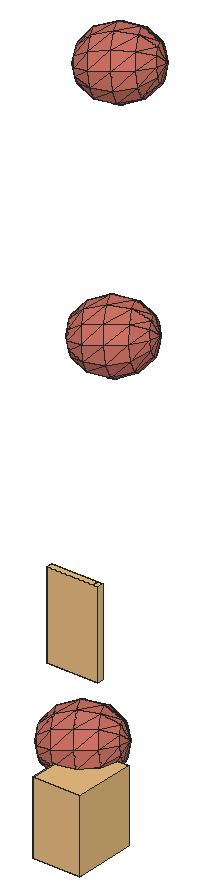
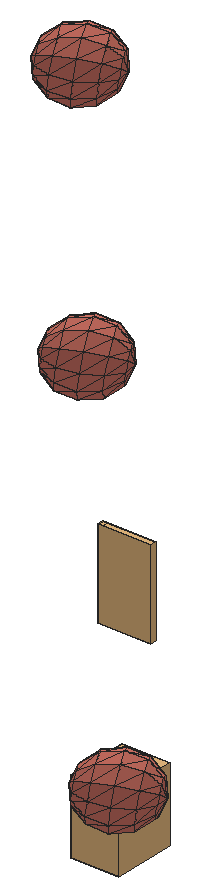
# SketchUp Ruby script. Lengths in inches.
U = 1.inch
M = Sketchup.active_model
def pt(a) = Geom::Point3d.new(a.map { |v| v * U })
def face(e, loops, mat)
  f = e.add_face(loops[0].map { |a| pt(a) })
  loops[1..].each { |l| e.add_face(l.map { |a| pt(a) }).erase! }
  f.material = f.back_material = mat if mat
  f
end
# faces: each face lists its corners as indices into pts; further lists are holes
def faces(e, pts, list, mat = nil) = list.each { |f| face(e, (f[0].is_a?(Array) ? f : [f]).map { |l| l.map { |i| pts[i] } }, mat) }
# xy, xz, yz: faces in a plane at the given z, y or x. An outline is a flat list of corners, or four numbers for a rectangle; further outlines are holes
def ring(l) = l.size == 4 ? [[l[0], l[1]], [l[2], l[1]], [l[2], l[3]], [l[0], l[3]]] : l.each_slice(2).to_a
def flat(e, list, mat, &to3) = list.each { |f| face(e, (f[0].is_a?(Array) ? f : [f]).map { |l| ring(l).map { |u, v| to3.(u, v) } }, mat) }
def xy(e, z, list, mat = nil) = flat(e, list, mat) { |x, y| [x, y, z] }
def xz(e, y, list, mat = nil) = flat(e, list, mat) { |x, z| [x, y, z] }
def yz(e, x, list, mat = nil) = flat(e, list, mat) { |y, z| [x, y, z] }
def lines(e, pts, list) = list.each { |a, b| e.add_line(pt(pts[a]), pt(pts[b])) }
# prism: a flat outline (further loops are holes) pulled along v
def prism(e, loops, v, mat = nil)
  f = face(e, loops, mat); d = Geom::Vector3d.new(v.map { |x| x * U })
  f.pushpull(f.normal.samedirection?(d) ? d.length : -d.length)
end
def box(e, o, s, mat = nil) = prism(e, [[o, [o[0] + s[0], o[1], o[2]], [o[0] + s[0], o[1] + s[1], o[2]], [o[0], o[1] + s[1], o[2]]]], [0, 0, s[2]], mat)
def at(x, y, z, deg = 0) = Geom::Transformation.translation(pt([x, y, z])) * Geom::Transformation.rotation(ORIGIN, Z_AXIS, deg.degrees)
def axes(o, x, y, z) = Geom::Transformation.new([*x, 0, *y, 0, *z, 0, *pt(o).to_a, 1])
def part(name) = M.definitions.add(name)
# library, detail: a bought-in or finely detailed component or shape, given as its bounding box
def library(name, o, s) = part(name).tap { |d| box(d.entities, o, s) }
def detail(e, o, s) = box(e.add_group.entities, o, s)
def put(e, d, t, mat = nil) = e.add_instance(d, t).tap { |i| i.material = mat if mat }
def group(e, t, mat = nil) = e.add_group.tap { |g| g.transformation = t; g.material = mat if mat }.entities
root = M.entities
M.materials.add("green").color = [174, 139, 102]
M.materials.add("vio").color = [206, 114, 100]
c1 = part("3DGeom~236_Defintion")
p = [[-0.24,-111.46,-482.47],[-247.71,40.8125,-431.68],[-3.37,-2.64,-500],[241.88,-45.39,-434.35],[50.53,96.35,-484.34],[-154.36,212.27,-404.56],
  [147.01,158.99,-439.69],[12.76,320.76,-327.23],[59.09,-200.9375,-436.46],[-242.29,-147.66,-401.32],[260.24,168.49,-378.02],[208.87,337.23,-220.41],
  [208.87,337.23,-220.41],[-139.53,-302.65,-321.625],[158.71,-247.11,-374.29],[271.93,-237.61,-312.62],[368.42,-174.96,-267.97],[422.32,-75.98,-252.31],
  [419.18,32.84,-269.83],[359.86,122.32,-315.85],[-242.29,-147.66,-401.32],[-425.68,73.33,-247.69],[-247.71,40.8125,-431.68],[-425.68,73.33,-247.69],
  [-317.89,271.31,-216.37],[-317.89,271.31,-216.37],[-154.36,212.27,-404.56],[-317.89,271.31,-216.37],[-124.92,396.59,-127.08],[-154.36,212.27,-404.56],
  [12.76,320.76,-327.23],[-139.53,-302.65,-321.625],[-419.42,-144.29,-212.64],[-242.29,-147.66,-401.32],[-242.29,-147.66,-401.32],[-425.68,73.33,-247.69],
  [260.24,168.49,-378.02],[381.41,257.26,-112.72],[359.86,122.32,-315.85],[260.24,168.49,-378.02],[208.87,337.23,-220.41],[33.01,-382.62,-213.94],
  [271.93,-237.61,-312.62],[33.01,-382.62,-213.94],[158.71,-247.11,-374.29],[12.76,320.76,-327.23],[101.53,415.61,-3.73],[12.76,320.76,-327.23],
  [208.87,337.23,-220.41],[33.01,-382.62,-213.94],[-300.77,-323.26,-120.61],[-139.53,-302.65,-321.625],[-139.53,-302.65,-321.625],[-300.77,-323.26,-120.61],
  [359.86,122.32,-315.85],[484.17,102.27,-33.02],[419.18,32.84,-269.83],[359.86,122.32,-315.85],[271.93,-237.61,-312.62],[229.12,-366.15,-107.12],
  [33.01,-382.62,-213.94],[368.42,-174.96,-267.97],[229.12,-366.15,-107.12],[271.93,-237.61,-312.62],[419.18,32.84,-269.83],[489.59,-86.2,-2.67],
  [419.18,32.84,-269.83],[422.32,-75.98,-252.31],[368.42,-174.96,-267.97],[396.24,-257.66,-29.79],[229.12,-366.15,-107.12],[422.32,-75.98,-252.31],
  [368.42,-174.96,-267.97],[422.32,-75.98,-252.31],[-489.59,86.2,2.67],[-425.68,73.33,-247.69],[-425.68,73.33,-247.69],[-396.24,257.66,29.79],
  [-425.68,73.33,-247.69],[-396.24,257.66,29.79],[-317.89,271.31,-216.37],[208.87,337.23,-220.41],[300.77,323.26,120.61],[381.41,257.26,-112.72],
  [208.87,337.23,-220.41],[300.77,323.26,120.61],[-396.24,257.66,29.79],[-229.12,366.15,107.12],[33.01,-382.62,-213.94],[-101.53,-415.61,3.73],
  [-300.77,-323.26,-120.61],[33.01,-382.62,-213.94],[-484.17,-102.27,33.02],[-33.01,382.62,213.94],[-381.41,-257.26,112.72],[-300.77,-323.26,-120.61],
  [-381.41,-257.26,112.72],[419.42,144.29,212.64],[300.77,323.26,120.61],[124.92,-396.59,127.08],[396.24,-257.66,-29.79],[425.68,-73.33,247.69],
  [396.24,-257.66,-29.79],[317.89,-271.31,216.37],[317.89,-271.31,216.37],[139.53,302.65,321.625],[139.53,302.65,321.625],[300.77,323.26,120.61],
  [-422.32,75.98,252.31],[-368.42,174.96,267.97],[-396.24,257.66,29.79],[-208.87,-337.23,220.41],[-381.41,-257.26,112.72],[-396.24,257.66,29.79],
  [-271.93,237.61,312.62],[-396.24,257.66,29.79],[-271.93,237.61,312.62],[-229.12,366.15,107.12],[-419.18,-32.84,269.83],[-271.93,237.61,312.62],
  [-158.71,247.11,374.29],[-158.71,247.11,374.29],[-208.87,-337.23,220.41],[-359.86,-122.32,315.85],[242.29,147.66,401.32],[139.53,302.65,321.625],
  [-12.76,-320.76,327.23],[317.89,-271.31,216.37],[247.71,-40.8125,431.68],[247.71,-40.8125,431.68],[-33.01,382.62,213.94],[-158.71,247.11,374.29],
  [-59.09,200.94,436.46],[-33.01,382.62,213.94],[139.53,302.65,321.625],[317.89,-271.31,216.37],[154.36,-212.27,404.56],[425.68,-73.33,247.69],
  [154.36,-212.27,404.56],[317.89,-271.31,216.37],[-208.87,-337.23,220.41],[-260.24,-168.49,378.02],[-12.76,-320.76,327.23],[-260.24,-168.49,378.02],
  [-208.87,-337.23,220.41],[425.68,-73.33,247.69],[247.71,-40.8125,431.68],[-422.32,75.98,252.31],[-419.18,-32.84,269.83],[-241.88,45.39,434.35],
  [-368.42,174.96,267.97],[-422.32,75.98,252.31],[-271.93,237.61,312.62],[-368.42,174.96,267.97],[-419.18,-32.84,269.83],[-359.86,-122.32,315.85],
  [-271.93,237.61,312.62],[-359.86,-122.32,315.85],[-260.24,-168.49,378.02],[139.53,302.65,321.625],[0.24,111.46,482.47],[139.53,302.65,321.625],
  [242.29,147.66,401.32],[-12.76,-320.76,327.23],[-147.01,-158.99,439.69],[-260.24,-168.49,378.02],[-12.76,-320.76,327.23],[-260.24,-168.49,378.02],
  [242.29,147.66,401.32],[3.37,2.64,500],[242.29,147.66,401.32],[-50.53,-96.35,484.34]]
faces(c1.entities,p,[[0,1,2],[0,2,3],[2,4,3],[2,1,5],[2,5,4],[4,6,3],[4,5,7],[4,7,6],
  [8,9,0],[8,0,3],[0,9,1],[6,10,3],[6,7,11],[6,12,10],[8,13,9],[14,13,8],
  [14,8,3],[15,14,3],[16,15,3],[17,16,3],[18,17,3],[19,18,3],[10,19,3],[20,21,22],
  [1,23,24],[1,25,5],[26,27,28],[29,28,30],[31,32,33],[34,32,35],[36,37,38],[39,40,37],
  [14,41,13],[42,43,44],[45,28,46],[47,46,48],[49,50,51],[52,53,32],[54,55,56],[57,37,55],
  [58,59,60],[61,62,63],[64,55,65],[66,65,67],[68,69,70],[71,69,72],[73,65,69],[32,74,75],
  [76,74,77],[78,79,80],[81,82,83],[84,46,85],[27,86,87],[27,87,28],[88,89,90],[59,89,91],
  [53,92,32],[32,92,74],[28,87,93],[28,93,46],[89,94,95],[53,96,92],[37,97,55],[37,98,97],
  [59,99,89],[100,99,59],[55,101,65],[55,97,101],[102,103,99],[65,104,69],[46,93,105],[46,106,107],
  [65,101,104],[92,108,74],[74,108,109],[74,109,110],[89,111,112],[99,111,89],[113,109,114],[115,116,117],
  [96,118,92],[92,118,108],[87,119,120],[87,121,93],[122,123,96],[96,123,118],[98,124,97],[98,125,124],
  [99,126,111],[127,126,99],[97,128,101],[97,124,129],[130,131,132],[133,132,134],[135,136,126],[137,138,139],
  [140,141,123],[142,143,144],[145,146,138],[147,148,149],[150,151,149],[152,153,149],[154,155,149],[131,156,149],
  [157,158,149],[159,132,160],[161,160,162],[163,164,165],[138,164,166],[132,131,149],[167,164,149],[168,169,146],
  [170,160,169],[138,171,164],[146,171,138],[146,169,171],[164,171,149],[171,169,149],[169,160,149],[160,132,149]],"vio")
c2 = library("3DGeom~148_Defintion",[-424.75,-500,-323.76],[849.5,1000,647.52])
c3 = part("3DGeom~149_Defintion")
p = [[-419.66,479.4,-302.56],[-386.2,481.32,-323.76],[-405.55,478.95,-317.48],[-419.66,479.4,-302.56],[-366.78,485.875,-319.73],[-386.2,481.32,-323.76],
  [-419.66,479.4,-302.56],[-352.51,491.39,-306.47],[-366.78,485.875,-319.73],[-419.66,479.4,-302.56],[-347.21,496.4,-287.52],[-352.51,491.39,-306.47],
  [-419.66,479.4,-302.56],[-424.75,482.55,-283.01],[-419.44,487.56,-264.0625],[-419.66,479.4,-302.56],[-366.41,500,-253.05],[-352.3,499.55,-267.97],
  [-419.66,479.4,-302.56],[-352.3,499.55,-267.97],[-347.21,496.4,-287.52],[-419.66,479.4,-302.56],[-405.17,493.08,-250.79],[-385.76,497.63,-246.76],
  [-419.66,479.4,-302.56],[-385.76,497.63,-246.76],[-366.41,500,-253.05],[-419.66,479.4,-302.56],[-419.44,487.56,-264.0625],[-405.17,493.08,-250.79],
  [368.25,-500,278.25],[381.22,-498.52,262.42],[397.44,-490.86,253.62],[422.57,-466.35,264.06],[368.25,-500,278.25],[397.44,-490.86,253.62],
  [422.57,-466.35,264.06],[397.44,-490.86,253.62],[412.58,-479.09,254.22],[418.52,-450.97,299.13],[368.25,-500,278.25],[422.57,-466.35,264.06],
  [422.57,-466.35,264.06],[424.75,-456.06,280.5],[368.25,-500,278.25],[364.2,-484.62,313.32],[362.02,-494.91,296.88],[364.2,-484.62,313.32],
  [368.25,-500,278.25],[389.33,-460.11,323.76],[389.33,-460.11,323.76],[368.25,-500,278.25],[389.33,-460.11,323.76],[405.55,-452.45,314.97],
  [364.2,-484.62,313.32],[389.33,-460.11,323.76],[374.19,-471.88,323.16]]
faces(c3.entities,p,[[0,1,2],[3,4,5],[6,7,8],[9,10,11],[12,13,14],[15,16,17],[18,19,20],[21,22,23],
  [24,25,26],[27,28,29],[30,31,32],[33,34,35],[36,37,38],[39,40,41],[39,42,43],[44,45,46],
  [47,48,49],[50,51,39],[52,39,53],[54,55,56]],"green")
c4 = part("3DGeom~234_Defintion")
p = [[-0.24,-111.46,-482.48],[-247.71,40.8125,-431.68],[-3.37,-2.64,-500],[241.88,-45.39,-434.35],[50.53,96.35,-484.34],[-154.36,212.27,-404.56],
  [147.01,158.99,-439.69],[12.76,320.76,-327.23],[59.09,-200.9375,-436.46],[-242.29,-147.66,-401.33],[260.24,168.49,-378.02],[208.87,337.23,-220.41],
  [208.87,337.23,-220.41],[-139.53,-302.65,-321.625],[158.71,-247.11,-374.29],[271.93,-237.61,-312.62],[368.42,-174.96,-267.97],[422.32,-75.98,-252.31],
  [419.18,32.84,-269.83],[359.86,122.32,-315.85],[-242.29,-147.66,-401.33],[-425.69,73.33,-247.69],[-247.71,40.8125,-431.68],[-425.69,73.33,-247.69],
  [-317.89,271.31,-216.375],[-317.89,271.31,-216.375],[-154.36,212.27,-404.56],[-317.89,271.31,-216.375],[-124.92,396.59,-127.08],[-154.36,212.27,-404.56],
  [12.76,320.76,-327.23],[-139.53,-302.65,-321.625],[-419.42,-144.29,-212.64],[-242.29,-147.66,-401.33],[-242.29,-147.66,-401.33],[-425.69,73.33,-247.69],
  [260.24,168.49,-378.02],[381.41,257.26,-112.72],[359.86,122.32,-315.85],[260.24,168.49,-378.02],[208.87,337.23,-220.41],[33.01,-382.62,-213.94],
  [271.93,-237.61,-312.62],[33.01,-382.62,-213.94],[158.71,-247.11,-374.29],[12.76,320.76,-327.23],[101.53,415.61,-3.73],[12.76,320.76,-327.23],
  [208.87,337.23,-220.41],[33.01,-382.62,-213.94],[-300.77,-323.26,-120.61],[-139.53,-302.65,-321.625],[-139.53,-302.65,-321.625],[-300.77,-323.26,-120.61],
  [359.86,122.32,-315.85],[484.17,102.27,-33.02],[419.18,32.84,-269.83],[359.86,122.32,-315.85],[271.93,-237.61,-312.62],[229.12,-366.15,-107.12],
  [33.01,-382.62,-213.94],[368.42,-174.96,-267.97],[229.12,-366.15,-107.12],[271.93,-237.61,-312.62],[419.18,32.84,-269.83],[489.59,-86.2,-2.67],
  [419.18,32.84,-269.83],[422.32,-75.98,-252.31],[368.42,-174.96,-267.97],[396.24,-257.66,-29.79],[229.12,-366.15,-107.12],[422.32,-75.98,-252.31],
  [368.42,-174.96,-267.97],[422.32,-75.98,-252.31],[-489.59,86.2,2.67],[-425.69,73.33,-247.69],[-425.69,73.33,-247.69],[-396.24,257.66,29.79],
  [-425.69,73.33,-247.69],[-396.24,257.66,29.79],[-317.89,271.31,-216.375],[208.87,337.23,-220.41],[300.77,323.26,120.61],[381.41,257.26,-112.72],
  [208.87,337.23,-220.41],[300.77,323.26,120.61],[-396.24,257.66,29.79],[-229.12,366.15,107.12],[33.01,-382.62,-213.94],[-101.53,-415.61,3.73],
  [-300.77,-323.26,-120.61],[33.01,-382.62,-213.94],[-484.17,-102.27,33.02],[-33.01,382.62,213.94],[-381.41,-257.26,112.72],[-300.77,-323.26,-120.61],
  [-381.41,-257.26,112.72],[419.42,144.29,212.64],[300.77,323.26,120.61],[124.92,-396.59,127.08],[396.24,-257.66,-29.79],[425.69,-73.33,247.69],
  [396.24,-257.66,-29.79],[317.89,-271.31,216.375],[317.89,-271.31,216.375],[139.53,302.65,321.625],[139.53,302.65,321.625],[300.77,323.26,120.61],
  [-422.32,75.98,252.31],[-368.42,174.96,267.97],[-396.24,257.66,29.79],[-208.87,-337.23,220.41],[-381.41,-257.26,112.72],[-396.24,257.66,29.79],
  [-271.93,237.61,312.62],[-396.24,257.66,29.79],[-271.93,237.61,312.62],[-229.12,366.15,107.12],[-419.18,-32.84,269.83],[-271.93,237.61,312.62],
  [-158.71,247.11,374.29],[-158.71,247.11,374.29],[-208.87,-337.23,220.41],[-359.86,-122.32,315.85],[242.29,147.66,401.33],[139.53,302.65,321.625],
  [-12.76,-320.76,327.23],[317.89,-271.31,216.375],[247.71,-40.8125,431.68],[247.71,-40.8125,431.68],[-33.01,382.62,213.94],[-158.71,247.11,374.29],
  [-59.09,200.94,436.46],[-33.01,382.62,213.94],[139.53,302.65,321.625],[317.89,-271.31,216.375],[154.36,-212.27,404.56],[425.69,-73.33,247.69],
  [154.36,-212.27,404.56],[317.89,-271.31,216.375],[-208.87,-337.23,220.41],[-260.24,-168.49,378.02],[-12.76,-320.76,327.23],[-260.24,-168.49,378.02],
  [-208.87,-337.23,220.41],[425.69,-73.33,247.69],[247.71,-40.8125,431.68],[-422.32,75.98,252.31],[-419.18,-32.84,269.83],[-241.88,45.39,434.35],
  [-368.42,174.96,267.97],[-422.32,75.98,252.31],[-271.93,237.61,312.62],[-368.42,174.96,267.97],[-419.18,-32.84,269.83],[-359.86,-122.32,315.85],
  [-271.93,237.61,312.62],[-359.86,-122.32,315.85],[-260.24,-168.49,378.02],[139.53,302.65,321.625],[0.24,111.46,482.48],[139.53,302.65,321.625],
  [242.29,147.66,401.33],[-12.76,-320.76,327.23],[-147.01,-158.99,439.69],[-260.24,-168.49,378.02],[-12.76,-320.76,327.23],[-260.24,-168.49,378.02],
  [242.29,147.66,401.33],[3.37,2.64,500],[242.29,147.66,401.33],[-50.53,-96.35,484.34]]
faces(c4.entities,p,[[0,1,2],[0,2,3],[2,4,3],[2,1,5],[2,5,4],[4,6,3],[4,5,7],[4,7,6],
  [8,9,0],[8,0,3],[0,9,1],[6,10,3],[6,7,11],[6,12,10],[8,13,9],[14,13,8],
  [14,8,3],[15,14,3],[16,15,3],[17,16,3],[18,17,3],[19,18,3],[10,19,3],[20,21,22],
  [1,23,24],[1,25,5],[26,27,28],[29,28,30],[31,32,33],[34,32,35],[36,37,38],[39,40,37],
  [14,41,13],[42,43,44],[45,28,46],[47,46,48],[49,50,51],[52,53,32],[54,55,56],[57,37,55],
  [58,59,60],[61,62,63],[64,55,65],[66,65,67],[68,69,70],[71,69,72],[73,65,69],[32,74,75],
  [76,74,77],[78,79,80],[81,82,83],[84,46,85],[27,86,87],[27,87,28],[88,89,90],[59,89,91],
  [53,92,32],[32,92,74],[28,87,93],[28,93,46],[89,94,95],[53,96,92],[37,97,55],[37,98,97],
  [59,99,89],[100,99,59],[55,101,65],[55,97,101],[102,103,99],[65,104,69],[46,93,105],[46,106,107],
  [65,101,104],[92,108,74],[74,108,109],[74,109,110],[89,111,112],[99,111,89],[113,109,114],[115,116,117],
  [96,118,92],[92,118,108],[87,119,120],[87,121,93],[122,123,96],[96,123,118],[98,124,97],[98,125,124],
  [99,126,111],[127,126,99],[97,128,101],[97,124,129],[130,131,132],[133,132,134],[135,136,126],[137,138,139],
  [140,141,123],[142,143,144],[145,146,138],[147,148,149],[150,151,149],[152,153,149],[154,155,149],[131,156,149],
  [157,158,149],[159,132,160],[161,160,162],[163,164,165],[138,164,166],[132,131,149],[167,164,149],[168,169,146],
  [170,160,169],[138,171,164],[146,171,138],[146,169,171],[164,171,149],[171,169,149],[169,160,149],[160,132,149]],"vio")
c5 = library("3DGeom~127_Defintion",[-35.65,-500,-298.26],[71.3,1000,596.52])
c6 = part("3DGeom~128_Defintion")
p = [[1.79,-469.7,-298.26],[1.7,-500,-240.6],[-27.6,-477.32,-283.92],[31.13,-477.23,-283.76],[1.7,-500,-240.6],[1.79,-469.7,-298.26],
  [1.79,-469.7,-298.26],[-27.6,-477.32,-283.92],[-15.17,-471.75,-294.44],[31.13,-477.23,-283.76],[1.79,-469.7,-298.26],[18.74,-471.7,-294.35],
  [-27.6,-477.32,-283.92],[1.7,-500,-240.6],[-27.65,-492.47,-255.09],[-27.6,-477.32,-283.92],[-27.65,-492.47,-255.09],[-32.17,-484.9,-269.52],
  [31.09,-492.38,-254.93],[1.7,-500,-240.6],[31.13,-477.23,-283.76],[31.09,-492.38,-254.93],[31.13,-477.23,-283.76],[35.65,-484.8,-269.34],
  [1.7,-500,-240.6],[-15.25,-498,-244.5],[-27.65,-492.47,-255.09],[1.7,-500,-240.6],[31.09,-492.38,-254.93],[18.66,-497.94,-244.41],
  [-1.83,497.78,298.26],[-1.65,500,230.49],[-18.62,499.82,234.98],[-1.83,497.78,298.26],[15.29,499.875,235.07],[-1.65,500,230.49],
  [-1.83,497.78,298.26],[-18.62,499.82,234.98],[-31.0625,499.4,247.35],[-1.83,497.78,298.26],[27.67,499.49,247.51],[15.29,499.875,235.07],
  [-1.83,497.78,298.26],[-31.0625,499.4,247.35],[-35.65,498.84,264.28],[-1.83,497.78,298.26],[32.17,498.94,264.47],[27.67,499.49,247.51],
  [-1.83,497.78,298.26],[-35.65,498.84,264.28],[-31.15,498.29,281.24],[-1.83,497.78,298.26],[27.58,498.375,281.4],[32.17,498.94,264.47],
  [-1.83,497.78,298.26],[-31.15,498.29,281.24],[-18.77,497.9,293.67],[-1.83,497.78,298.26],[15.14,497.95,293.77],[27.58,498.375,281.4]]
faces(c6.entities,p,[[0,1,2],[3,4,5],[6,7,8],[9,10,11],[12,13,14],[15,16,17],[18,19,20],[21,22,23],
  [24,25,26],[27,28,29],[30,31,32],[33,34,35],[36,37,38],[39,40,41],[42,43,44],[45,46,47],
  [48,49,50],[51,52,53],[54,55,56],[57,58,59]],"green")
c7 = part("3DGeom~232_Defintion")
p = [[-0.24,-111.46,-482.48],[-247.71,40.8125,-431.68],[-3.37,-2.64,-500],[241.88,-45.39,-434.35],[50.53,96.35,-484.34],[-154.36,212.27,-404.56],
  [147.01,158.99,-439.69],[12.76,320.76,-327.23],[59.09,-200.9375,-436.46],[-242.29,-147.66,-401.33],[260.24,168.49,-378.02],[208.87,337.23,-220.41],
  [208.87,337.23,-220.41],[-139.53,-302.65,-321.625],[158.71,-247.11,-374.29],[271.93,-237.61,-312.62],[368.42,-174.96,-267.97],[422.32,-75.98,-252.31],
  [419.18,32.84,-269.83],[359.86,122.32,-315.85],[-242.29,-147.66,-401.33],[-425.69,73.33,-247.69],[-247.71,40.8125,-431.68],[-425.69,73.33,-247.69],
  [-317.89,271.31,-216.375],[-317.89,271.31,-216.375],[-154.36,212.27,-404.56],[-317.89,271.31,-216.375],[-124.92,396.59,-127.08],[-154.36,212.27,-404.56],
  [12.76,320.76,-327.23],[-139.53,-302.65,-321.625],[-419.42,-144.29,-212.64],[-242.29,-147.66,-401.33],[-242.29,-147.66,-401.33],[-425.69,73.33,-247.69],
  [260.24,168.49,-378.02],[381.41,257.26,-112.72],[359.86,122.32,-315.85],[260.24,168.49,-378.02],[208.87,337.23,-220.41],[33.01,-382.62,-213.94],
  [271.93,-237.61,-312.62],[33.01,-382.62,-213.94],[158.71,-247.11,-374.29],[12.76,320.76,-327.23],[101.53,415.61,-3.73],[12.76,320.76,-327.23],
  [208.87,337.23,-220.41],[33.01,-382.62,-213.94],[-300.77,-323.26,-120.61],[-139.53,-302.65,-321.625],[-139.53,-302.65,-321.625],[-300.77,-323.26,-120.61],
  [359.86,122.32,-315.85],[484.17,102.27,-33.02],[419.18,32.84,-269.83],[359.86,122.32,-315.85],[271.93,-237.61,-312.62],[229.12,-366.15,-107.12],
  [33.01,-382.62,-213.94],[368.42,-174.96,-267.97],[229.12,-366.15,-107.12],[271.93,-237.61,-312.62],[419.18,32.84,-269.83],[489.59,-86.2,-2.67],
  [419.18,32.84,-269.83],[422.32,-75.98,-252.31],[368.42,-174.96,-267.97],[396.24,-257.66,-29.79],[229.12,-366.15,-107.12],[422.32,-75.98,-252.31],
  [368.42,-174.96,-267.97],[422.32,-75.98,-252.31],[-489.59,86.2,2.67],[-425.69,73.33,-247.69],[-425.69,73.33,-247.69],[-396.24,257.66,29.79],
  [-425.69,73.33,-247.69],[-396.24,257.66,29.79],[-317.89,271.31,-216.375],[208.87,337.23,-220.41],[300.77,323.26,120.61],[381.41,257.26,-112.72],
  [208.87,337.23,-220.41],[300.77,323.26,120.61],[-396.24,257.66,29.79],[-229.12,366.15,107.12],[33.01,-382.62,-213.94],[-101.53,-415.61,3.73],
  [-300.77,-323.26,-120.61],[33.01,-382.62,-213.94],[-484.17,-102.27,33.02],[-33.01,382.62,213.94],[-381.41,-257.26,112.72],[-300.77,-323.26,-120.61],
  [-381.41,-257.26,112.72],[419.42,144.29,212.64],[300.77,323.26,120.61],[124.92,-396.59,127.08],[396.24,-257.66,-29.79],[425.69,-73.33,247.69],
  [396.24,-257.66,-29.79],[317.89,-271.31,216.375],[317.89,-271.31,216.375],[139.53,302.65,321.625],[139.53,302.65,321.625],[300.77,323.26,120.61],
  [-422.32,75.98,252.31],[-368.42,174.96,267.97],[-396.24,257.66,29.79],[-208.87,-337.23,220.41],[-381.41,-257.26,112.72],[-396.24,257.66,29.79],
  [-271.93,237.61,312.62],[-396.24,257.66,29.79],[-271.93,237.61,312.62],[-229.12,366.15,107.12],[-419.18,-32.84,269.83],[-271.93,237.61,312.62],
  [-158.71,247.11,374.29],[-158.71,247.11,374.29],[-208.87,-337.23,220.41],[-359.86,-122.32,315.85],[242.29,147.66,401.33],[139.53,302.65,321.625],
  [-12.76,-320.76,327.23],[317.89,-271.31,216.375],[247.71,-40.8125,431.68],[247.71,-40.8125,431.68],[-33.01,382.62,213.94],[-158.71,247.11,374.29],
  [-59.09,200.94,436.46],[-33.01,382.62,213.94],[139.53,302.65,321.625],[317.89,-271.31,216.375],[154.36,-212.27,404.56],[425.69,-73.33,247.69],
  [154.36,-212.27,404.56],[317.89,-271.31,216.375],[-208.87,-337.23,220.41],[-260.24,-168.49,378.02],[-12.76,-320.76,327.23],[-260.24,-168.49,378.02],
  [-208.87,-337.23,220.41],[425.69,-73.33,247.69],[247.71,-40.8125,431.68],[-422.32,75.98,252.31],[-419.18,-32.84,269.83],[-241.88,45.39,434.35],
  [-368.42,174.96,267.97],[-422.32,75.98,252.31],[-271.93,237.61,312.62],[-368.42,174.96,267.97],[-419.18,-32.84,269.83],[-359.86,-122.32,315.85],
  [-271.93,237.61,312.62],[-359.86,-122.32,315.85],[-260.24,-168.49,378.02],[139.53,302.65,321.625],[0.24,111.46,482.48],[139.53,302.65,321.625],
  [242.29,147.66,401.33],[-12.76,-320.76,327.23],[-147.01,-158.99,439.69],[-260.24,-168.49,378.02],[-12.76,-320.76,327.23],[-260.24,-168.49,378.02],
  [242.29,147.66,401.33],[3.37,2.64,500],[242.29,147.66,401.33],[-50.53,-96.35,484.34]]
faces(c7.entities,p,[[0,1,2],[0,2,3],[2,4,3],[2,1,5],[2,5,4],[4,6,3],[4,5,7],[4,7,6],
  [8,9,0],[8,0,3],[0,9,1],[6,10,3],[6,7,11],[6,12,10],[8,13,9],[14,13,8],
  [14,8,3],[15,14,3],[16,15,3],[17,16,3],[18,17,3],[19,18,3],[10,19,3],[20,21,22],
  [1,23,24],[1,25,5],[26,27,28],[29,28,30],[31,32,33],[34,32,35],[36,37,38],[39,40,37],
  [14,41,13],[42,43,44],[45,28,46],[47,46,48],[49,50,51],[52,53,32],[54,55,56],[57,37,55],
  [58,59,60],[61,62,63],[64,55,65],[66,65,67],[68,69,70],[71,69,72],[73,65,69],[32,74,75],
  [76,74,77],[78,79,80],[81,82,83],[84,46,85],[27,86,87],[27,87,28],[88,89,90],[59,89,91],
  [53,92,32],[32,92,74],[28,87,93],[28,93,46],[89,94,95],[53,96,92],[37,97,55],[37,98,97],
  [59,99,89],[100,99,59],[55,101,65],[55,97,101],[102,103,99],[65,104,69],[46,93,105],[46,106,107],
  [65,101,104],[92,108,74],[74,108,109],[74,109,110],[89,111,112],[99,111,89],[113,109,114],[115,116,117],
  [96,118,92],[92,118,108],[87,119,120],[87,121,93],[122,123,96],[96,123,118],[98,124,97],[98,125,124],
  [99,126,111],[127,126,99],[97,128,101],[97,124,129],[130,131,132],[133,132,134],[135,136,126],[137,138,139],
  [140,141,123],[142,143,144],[145,146,138],[147,148,149],[150,151,149],[152,153,149],[154,155,149],[131,156,149],
  [157,158,149],[159,132,160],[161,160,162],[163,164,165],[138,164,166],[132,131,149],[167,164,149],[168,169,146],
  [170,160,169],[138,171,164],[146,171,138],[146,169,171],[164,171,149],[171,169,149],[169,160,149],[160,132,149]],"vio")
g1 = group(root,at(15.3125,38.42,26.21))
put(g1,c1,axes([-2.25,0.89,10.125],[0,0.00039,0],[0,0,-0.00039],[-0.00039,0,0]),"vio")
g2 = group(root,at(15.3125,38.42,26.21))
put(g2,c2,axes([-2.125,0.72,9.92],[0,0.00037,0],[0,0,-0.00037],[-0.00037,0,0]),"green")
put(g2,c3,axes([-2.125,0.72,9.92],[0,0.00037,0],[0,0,-0.00037],[-0.00037,0,0]),"green")
g3 = group(root,at(15.3125,38.42,26.21))
put(g3,c4,axes([-2.11,0.91,12.02],[0,0.00039,0],[0,0,-0.00039],[-0.00039,0,0]),"vio")
g4 = group(root,at(15.3125,38.42,26.21))
put(g4,c5,axes([-2.06,0.6,10.86],[0,0.00044,0],[0,0,-0.00044],[-0.00044,0,0]),"green")
put(g4,c6,axes([-2.06,0.6,10.86],[0,0.00044,0],[0,0,-0.00044],[-0.00044,0,0]),"green")
g5 = group(root,at(15.3125,38.42,26.21))
put(g5,c7,axes([-2.06,0.89,13.3],[0,0.00039,0],[0,0,-0.00039],[-0.00039,0,0]),"vio")
